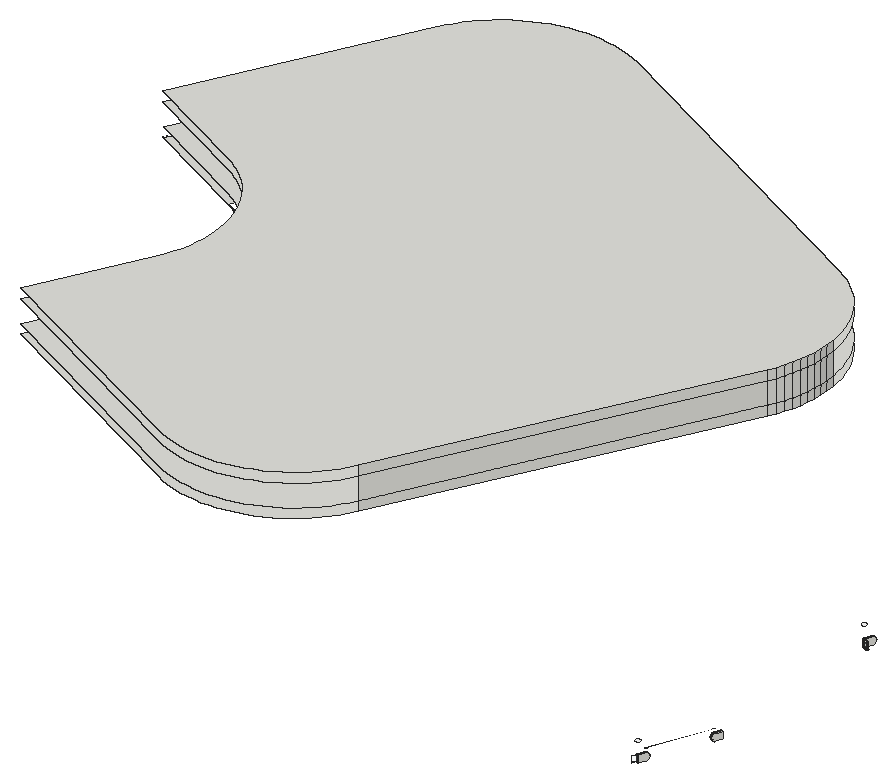
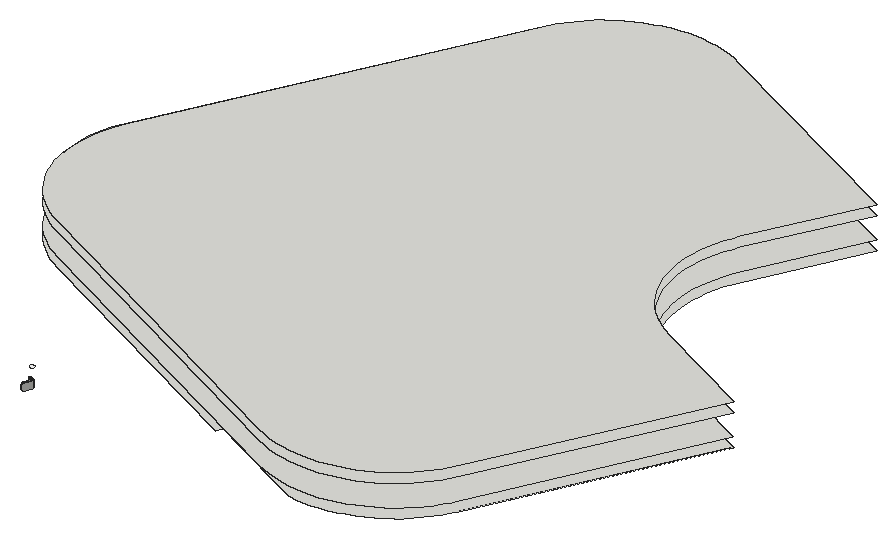
# SketchUp Ruby script. Lengths in inches.
U = 1.inch
M = Sketchup.active_model
def pt(a) = Geom::Point3d.new(a.map { |v| v * U })
def face(e, loops, mat)
  f = e.add_face(loops[0].map { |a| pt(a) })
  loops[1..].each { |l| e.add_face(l.map { |a| pt(a) }).erase! }
  f.material = f.back_material = mat if mat
  f
end
# faces: each face lists its corners as indices into pts; further lists are holes
def faces(e, pts, list, mat = nil) = list.each { |f| face(e, (f[0].is_a?(Array) ? f : [f]).map { |l| l.map { |i| pts[i] } }, mat) }
# xy, xz, yz: faces in a plane at the given z, y or x. An outline is a flat list of corners, or four numbers for a rectangle; further outlines are holes
def ring(l) = l.size == 4 ? [[l[0], l[1]], [l[2], l[1]], [l[2], l[3]], [l[0], l[3]]] : l.each_slice(2).to_a
def flat(e, list, mat, &to3) = list.each { |f| face(e, (f[0].is_a?(Array) ? f : [f]).map { |l| ring(l).map { |u, v| to3.(u, v) } }, mat) }
def xy(e, z, list, mat = nil) = flat(e, list, mat) { |x, y| [x, y, z] }
def xz(e, y, list, mat = nil) = flat(e, list, mat) { |x, z| [x, y, z] }
def yz(e, x, list, mat = nil) = flat(e, list, mat) { |y, z| [x, y, z] }
def lines(e, pts, list) = list.each { |a, b| e.add_line(pt(pts[a]), pt(pts[b])) }
# prism: a flat outline (further loops are holes) pulled along v
def prism(e, loops, v, mat = nil)
  f = face(e, loops, mat); d = Geom::Vector3d.new(v.map { |x| x * U })
  f.pushpull(f.normal.samedirection?(d) ? d.length : -d.length)
end
def box(e, o, s, mat = nil) = prism(e, [[o, [o[0] + s[0], o[1], o[2]], [o[0] + s[0], o[1] + s[1], o[2]], [o[0], o[1] + s[1], o[2]]]], [0, 0, s[2]], mat)
def at(x, y, z, deg = 0) = Geom::Transformation.translation(pt([x, y, z])) * Geom::Transformation.rotation(ORIGIN, Z_AXIS, deg.degrees)
def axes(o, x, y, z) = Geom::Transformation.new([*x, 0, *y, 0, *z, 0, *pt(o).to_a, 1])
def part(name) = M.definitions.add(name)
# library, detail: a bought-in or finely detailed component or shape, given as its bounding box
def library(name, o, s) = part(name).tap { |d| box(d.entities, o, s) }
def detail(e, o, s) = box(e.add_group.entities, o, s)
def put(e, d, t, mat = nil) = e.add_instance(d, t).tap { |i| i.material = mat if mat }
def group(e, t, mat = nil) = e.add_group.tap { |g| g.transformation = t; g.material = mat if mat }.entities
root = M.entities
M.materials.add("Glass_Safety_01").color = [204, 235, 244]
M.materials["Glass_Safety_01"].alpha = 0.1
M.materials.add("[Color_000]").color = [255, 255, 255]
xy(root,351.283,[[955.297,790.187,955.04,790.287,955.76,792.12,956.016,792.019],[954.857,790.359,954.6,790.46,954.605,790.472,954.611,790.484,954.86,790.366],[954.86,790.366,954.611,790.484,955.32,792.292,955.577,792.192],[962.61,810.093,962.354,810.194,963.074,812.026,963.33,811.925,962.671,810.249],[963.328,866.978,961.618,867.953,961.755,868.193,963.309,867.306,963.464,867.217],
  [963.562,867.388,963.406,867.477,962.17,868.183,962.28,868.437,963.698,867.627],[962.146,868.129,961.894,868.239,961.929,868.32,962.04,868.574,962.68,870.044,962.932,869.934,962.28,868.437,962.04,868.574,961.989,868.603,961.852,868.364,961.929,868.32,962.17,868.183],[962.17,868.183,961.929,868.32,962.04,868.574,962.28,868.437],[961.713,868.317,961.46,868.428,962.246,870.232,962.499,870.122],[961.929,868.32,961.852,868.364,961.989,868.603,962.04,868.574]])
xy(root,351.362,[[954.36,788.859,954.182,788.944,954.857,790.359,954.948,790.323,955.037,790.281],[955.04,790.287,954.948,790.323,954.86,790.366,955.433,791.825,955.616,791.753],[954.948,790.323,954.857,790.359,954.858,790.363,954.86,790.366],[963.122,867.412,961.755,868.193,961.803,868.278,961.894,868.239,961.929,868.32,963.22,867.583],[961.894,868.239,961.803,868.278,961.852,868.364,961.929,868.32],
  [961.803,868.278,961.713,868.317,962.342,869.761,962.522,869.683,961.929,868.32,961.852,868.364]],"Glass_Safety_01")
xy(root,353.33,[[954.36,788.859,955.037,790.281,954.948,790.323,954.857,790.359,954.182,788.944],[955.04,790.287,955.616,791.753,955.433,791.825,954.86,790.366,954.948,790.323],[954.948,790.323,954.86,790.366,954.858,790.363,954.857,790.359],[963.122,867.412,963.22,867.583,961.929,868.32,961.894,868.239,961.803,868.278,961.755,868.193],[961.894,868.239,961.929,868.32,961.852,868.364,961.803,868.278],
  [961.803,868.278,961.852,868.364,961.929,868.32,962.522,869.683,962.342,869.761,961.713,868.317]],"Glass_Safety_01")
xy(root,353.409,[[955.297,790.187,956.016,792.019,955.76,792.12,955.04,790.287],[954.857,790.359,954.86,790.366,954.611,790.484,954.605,790.472,954.6,790.46],[954.86,790.366,955.577,792.192,955.32,792.292,954.611,790.484],[962.61,810.093,962.671,810.249,963.33,811.925,963.074,812.026,962.354,810.194],[963.328,866.978,963.464,867.217,963.309,867.306,961.755,868.193,961.618,867.953],
  [962.146,868.129,962.17,868.183,961.929,868.32,961.852,868.364,961.989,868.603,962.04,868.574,962.28,868.437,962.932,869.934,962.68,870.044,962.04,868.574,961.929,868.32,961.894,868.239],[962.17,868.183,962.28,868.437,962.04,868.574,961.929,868.32],[961.713,868.317,962.499,870.122,962.246,870.232,961.46,868.428],[961.929,868.32,962.04,868.574,961.989,868.603,961.852,868.364]])
xy(root,354.511,[[955.76,792.12,962.671,810.249,955.577,792.192],[955.76,792.12,962.855,810.177,962.671,810.249]],"Glass_Safety_01")
xy(root,357.267,[[954.993,789.695,955.155,789.728,955.302,789.802,955.425,789.911,955.515,790.048,955.567,790.204,955.577,790.368,955.544,790.53,955.47,790.677,955.361,790.8,955.224,790.89,955.068,790.942,954.903,790.952,954.742,790.919,954.595,790.845,954.472,790.736,954.382,790.599,954.33,790.442,954.32,790.278,954.353,790.117,954.427,789.97,954.536,789.847,954.673,789.757,954.829,789.705],[961.848,867.65,962.009,867.683,962.157,867.757,962.279,867.866,962.37,868.003,962.422,868.159,962.432,868.323,962.399,868.484,962.325,868.631,962.216,868.754,962.079,868.845,961.922,868.897,961.758,868.907,961.597,868.873,961.45,868.8,961.327,868.691,961.237,868.553,961.185,868.397,961.175,868.233,961.208,868.072,961.282,867.925,961.391,867.802,961.528,867.712,961.684,867.66]],"[Color_000]")
xy(root,412.837,[[[862.815,738.526,860.46,738.588,858.115,738.805,855.788,739.175,853.491,739.695,851.232,740.366,849.022,741.182,846.871,742.141,777.884,775.639,793.609,808.023,794.568,810.175,795.384,812.385,796.054,814.643,796.575,816.941,796.945,819.267,797.161,821.613,797.224,823.968,797.132,826.322,796.887,828.665,796.489,830.987,795.94,833.278,795.243,835.528,794.399,837.728,793.414,839.868,792.291,841.938,791.035,843.931,789.651,845.838,788.145,847.65,786.524,849.359,784.795,850.959,782.965,852.442,781.042,853.803,779.034,855.034,776.949,856.132,744.842,871.723,776.516,936.952,776.255,937.079,744.581,871.849,744.565,871.857,776.004,936.603,776.255,937.079,777.102,938.6875,778.334,940.695,779.694,942.619,781.178,944.449,782.777,946.178,784.487,947.799,786.299,949.304,788.205,950.688,790.198,951.944,792.269,953.068,794.409,954.053,796.608,954.896,798.859,955.594,801.149,956.143,803.471,956.541,805.814,956.786,808.168,956.877,810.523,956.815,812.869,956.598,841.084,942.898,826.624,913.117,831.121,910.933,845.582,940.714,846.416,942.432,925.484,904.039,927.568,902.941,929.577,901.71,931.5,900.349,933.33,898.866,935.059,897.266,936.68,895.556,938.186,893.744,939.569,891.838,940.826,889.845,941.949,887.774,942.934,885.634,943.777,883.435,944.475,881.185,945.024,878.894,945.422,876.572,945.667,874.229,945.759,871.875,945.696,869.52,945.479,867.174,945.11,864.848,944.589,862.55,943.919,860.292,943.102,858.082,942.143,855.93,894.98,758.8,893.882,756.716,892.65,754.708,891.29,752.785,889.806,750.954,888.206,749.225,886.497,747.604,884.685,746.099,882.779,744.715,880.786,743.459,878.715,742.336,876.575,741.35,874.375,740.507,872.125,739.809,869.834,739.26,867.512,738.862,865.169,738.617],[780.848,854.239,812.287,918.985,808.388,920.878,776.949,856.132],[851.789,784.021,853.66,784.074,855.491,784.231,857.275,784.493,859.004,784.858,860.67,785.324,862.267,785.89,863.788,786.552,865.226,787.309,866.574,788.157,867.828,789.092,868.982,790.111,870.03,791.209,870.969,792.381,871.794,793.622,872.502,794.927,878.32,806.909,877.223,804.825,875.991,802.817,874.63,800.893,873.147,799.063,871.547,797.334,869.838,795.713,868.026,794.208,866.119,792.824,864.79,791.986,864.577,791.797,863.497,790.992,862.336,790.262,861.098,789.61,859.789,789.04,858.414,788.553,856.979,788.151,855.49,787.837,854.557,787.7,853.175,787.369,850.853,786.971,848.51,786.726,846.156,786.635,843.801,786.697,841.455,786.914,839.129,787.284,836.831,787.804,834.573,788.474,832.363,789.291,830.211,790.25,834.524,788.156,836.381,787.308,838.272,786.551,840.19,785.889,842.127,785.323,844.073,784.857,846.02,784.493,847.961,784.231,849.887,784.074]],[851.789,784.021,849.887,784.074,847.961,784.231,846.02,784.493,844.073,784.857,842.127,785.323,840.19,785.889,838.272,786.551,836.381,787.308,834.524,788.156,830.211,790.25,832.363,789.291,834.573,788.474,836.831,787.804,839.129,787.284,841.455,786.914,843.801,786.697,846.156,786.635,848.51,786.726,850.853,786.971,853.175,787.369,854.557,787.7,855.49,787.837,856.979,788.151,858.414,788.553,859.789,789.04,861.098,789.61,862.336,790.262,863.497,790.992,864.577,791.797,864.79,791.986,866.119,792.824,868.026,794.208,869.838,795.713,871.547,797.334,873.147,799.063,874.63,800.893,875.991,802.817,877.223,804.825,878.32,806.909,872.502,794.927,871.794,793.622,870.969,792.381,870.03,791.209,868.982,790.111,867.828,789.092,866.574,788.157,865.226,787.309,863.788,786.552,862.267,785.89,860.67,785.324,859.004,784.858,857.275,784.493,855.491,784.231,853.66,784.074]])
xy(root,415.758,[[862.815,738.526,860.46,738.588,858.115,738.805,855.788,739.175,853.491,739.695,851.232,740.366,849.022,741.182,846.871,742.141,777.884,775.639,793.609,808.023,794.568,810.175,795.384,812.385,796.054,814.643,796.575,816.941,796.945,819.267,797.161,821.613,797.224,823.968,797.132,826.322,796.887,828.665,796.489,830.987,795.94,833.278,795.243,835.528,794.399,837.728,793.414,839.868,792.291,841.938,791.035,843.931,789.651,845.838,788.145,847.65,786.524,849.359,784.795,850.959,782.965,852.442,781.042,853.803,779.034,855.034,776.949,856.132,744.842,871.723,776.516,936.952,776.255,937.079,777.102,938.6875,778.334,940.695,779.694,942.619,781.178,944.449,782.777,946.178,784.487,947.799,786.299,949.304,788.205,950.688,790.198,951.944,792.269,953.068,794.409,954.053,796.608,954.896,798.859,955.594,801.149,956.143,803.471,956.541,805.814,956.786,808.168,956.877,810.523,956.815,812.869,956.598,815.196,956.229,817.493,955.708,819.752,955.038,821.961,954.221,824.113,953.262,925.484,904.039,927.568,902.941,929.577,901.71,931.5,900.349,933.33,898.866,935.059,897.266,936.68,895.556,938.186,893.744,939.569,891.838,940.826,889.845,941.949,887.774,942.934,885.634,943.777,883.435,944.475,881.185,945.024,878.894,945.422,876.572,945.667,874.229,945.759,871.875,945.696,869.52,945.479,867.174,945.11,864.848,944.589,862.55,943.919,860.292,943.102,858.082,942.143,855.93,894.98,758.8,893.882,756.716,892.65,754.708,891.29,752.785,889.806,750.954,888.206,749.225,886.497,747.604,884.685,746.099,882.779,744.715,880.786,743.459,878.715,742.336,876.575,741.35,874.375,740.507,872.125,739.809,869.834,739.26,867.512,738.862,865.169,738.617]])
xy(root,422.51,[[862.815,738.526,860.46,738.588,858.115,738.805,855.788,739.175,853.491,739.695,851.232,740.366,849.022,741.182,846.871,742.141,777.884,775.639,793.609,808.023,794.568,810.175,795.384,812.385,796.054,814.643,796.575,816.941,796.945,819.267,797.161,821.613,797.224,823.968,797.132,826.322,796.887,828.665,796.489,830.987,795.94,833.278,795.243,835.528,794.399,837.728,793.414,839.868,792.291,841.938,791.035,843.931,789.651,845.838,788.145,847.65,786.524,849.359,784.795,850.959,782.965,852.442,781.042,853.803,779.034,855.034,776.949,856.132,744.565,871.857,776.004,936.603,777.102,938.6875,778.334,940.695,779.694,942.619,781.178,944.449,782.777,946.178,784.487,947.799,786.299,949.304,788.205,950.688,790.198,951.944,792.269,953.068,794.409,954.053,796.608,954.896,798.859,955.594,801.149,956.143,803.471,956.541,805.814,956.786,808.168,956.877,810.523,956.815,812.869,956.598,815.196,956.229,817.493,955.708,819.752,955.038,821.961,954.221,824.113,953.262,925.484,904.039,927.568,902.941,929.577,901.71,931.5,900.349,933.33,898.866,935.059,897.266,936.68,895.556,938.186,893.744,939.569,891.838,940.826,889.845,941.949,887.774,942.934,885.634,943.777,883.435,944.475,881.185,945.024,878.894,945.422,876.572,945.667,874.229,945.759,871.875,945.696,869.52,945.479,867.174,945.11,864.848,944.589,862.55,943.919,860.292,943.102,858.082,942.143,855.93,894.98,758.8,893.882,756.716,892.65,754.708,891.29,752.785,889.806,750.954,888.206,749.225,886.497,747.604,884.685,746.099,882.779,744.715,880.786,743.459,878.715,742.336,876.575,741.35,874.375,740.507,872.125,739.809,869.834,739.26,867.512,738.862,865.169,738.617]])
xy(root,425.526,[[862.815,738.526,865.169,738.617,867.512,738.862,869.834,739.26,872.125,739.809,874.375,740.507,876.575,741.35,878.715,742.336,880.786,743.459,882.779,744.715,884.685,746.099,886.497,747.604,888.206,749.225,889.806,750.954,891.29,752.785,892.65,754.708,893.882,756.716,894.98,758.8,942.143,855.93,943.102,858.082,943.919,860.292,944.589,862.55,945.11,864.848,945.479,867.174,945.696,869.52,945.759,871.875,945.667,874.229,945.422,876.572,945.024,878.894,944.475,881.185,943.777,883.435,942.934,885.634,941.949,887.774,940.826,889.845,939.569,891.838,938.186,893.744,936.68,895.556,935.059,897.266,933.33,898.866,931.5,900.349,929.577,901.71,927.568,902.941,925.484,904.039,824.113,953.262,821.961,954.221,819.752,955.038,817.493,955.708,815.196,956.229,812.869,956.598,810.523,956.815,808.168,956.877,805.814,956.786,803.471,956.541,801.149,956.143,798.859,955.594,796.608,954.896,794.409,954.053,792.269,953.068,790.198,951.944,788.205,950.688,786.299,949.304,784.487,947.799,782.777,946.178,781.178,944.449,779.694,942.619,778.334,940.695,777.102,938.6875,776.004,936.603,744.565,871.857,776.949,856.132,779.034,855.034,781.042,853.803,782.965,852.442,784.795,850.959,786.524,849.359,788.145,847.65,789.651,845.838,791.035,843.931,792.291,841.938,793.414,839.868,794.399,837.728,795.243,835.528,795.94,833.278,796.489,830.987,796.887,828.665,797.132,826.322,797.224,823.968,797.161,821.613,796.945,819.267,796.575,816.941,796.054,814.643,795.384,812.385,794.568,810.175,793.609,808.023,777.884,775.639,846.871,742.141,849.022,741.182,851.232,740.366,853.491,739.695,855.788,739.175,858.115,738.805,860.46,738.588]])
p = [[955.037,790.281,351.283],[955.037,790.281,351.362],[955.037,790.281,353.33],[955.037,790.281,353.409],[955.286,790.162,353.409],[955.286,790.162,351.283],
  [955.04,790.287,351.362],[955.04,790.287,351.283],[955.297,790.187,351.283],[955.297,790.187,353.409],[955.04,790.287,353.409],[955.04,790.287,353.33],
  [956.016,792.019,353.409],[956.016,792.019,351.283],[956.117,792.275,351.319],[956.211,792.513,351.425],[956.291,792.718,351.594],[956.353,792.876,351.814],
  [956.392,792.974,352.071],[956.405,793.008,352.346],[956.392,792.974,352.621],[956.353,792.876,352.877],[956.291,792.718,353.098],[956.211,792.513,353.267],
  [956.117,792.275,353.373],[955.76,792.12,353.409],[955.76,792.12,351.283],[955.616,791.753,351.362],[955.616,791.753,353.33],[954.857,790.359,351.283],
  [954.857,790.359,351.362],[954.857,790.359,353.33],[954.857,790.359,353.409],[954.6,790.46,353.409],[954.6,790.46,351.283],[954.86,790.366,351.362],
  [954.86,790.366,351.283],[954.611,790.484,351.283],[954.611,790.484,353.409],[954.86,790.366,353.409],[954.86,790.366,353.33],[955.577,792.192,351.283],
  [955.677,792.448,351.319],[955.771,792.686,351.425],[955.852,792.891,351.594],[955.913,793.048,351.814],[955.952,793.147,352.071],[955.965,793.181,352.346],
  [955.952,793.147,352.621],[955.913,793.048,352.877],[955.852,792.891,353.098],[955.771,792.686,353.267],[955.677,792.448,353.373],[955.577,792.192,353.409],
  [954.605,790.472,351.283],[954.605,790.472,353.409],[955.32,792.292,353.409],[955.421,792.548,353.373],[955.515,792.787,353.267],[955.595,792.992,353.098],
  [955.657,793.149,352.877],[955.696,793.248,352.621],[955.709,793.282,352.346],[955.696,793.248,352.071],[955.657,793.149,351.814],[955.595,792.992,351.594],
  [955.515,792.787,351.425],[955.421,792.548,351.319],[955.32,792.292,351.283],[955.86,792.376,351.319],[955.954,792.614,351.425],[956.035,792.819,351.594],
  [956.097,792.976,351.814],[956.135,793.075,352.071],[956.149,793.109,352.346],[956.135,793.075,352.621],[956.097,792.976,352.877],[956.035,792.819,353.098],
  [955.954,792.614,353.267],[955.86,792.376,353.373],[963.05,809.92,351.283],[963.765,811.74,351.283],[963.765,811.74,353.409],[963.05,809.92,353.409],
  [962.949,809.664,353.373],[962.856,809.426,353.267],[962.775,809.221,353.098],[962.713,809.064,352.877],[962.675,808.965,352.621],[962.661,808.931,352.346],
  [962.675,808.965,352.071],[962.713,809.064,351.814],[962.775,809.221,351.594],[962.856,809.426,351.425],[962.949,809.664,351.319],[962.855,810.177,353.409],
  [963.512,811.85,353.409],[963.512,811.85,353.33],[963.512,811.85,351.362],[963.512,811.85,351.283],[962.855,810.177,351.283],[962.794,810.021,351.283],
  [962.693,809.765,351.319],[962.599,809.527,351.425],[962.519,809.322,351.594],[962.457,809.164,351.814],[962.418,809.066,352.071],[962.405,809.032,352.346],
  [962.418,809.066,352.621],[962.457,809.164,352.877],[962.519,809.322,353.098],[962.599,809.527,353.267],[962.693,809.765,353.373],[962.794,810.021,353.409],
  [962.61,810.093,351.283],[962.671,810.249,351.283],[962.671,810.249,353.409],[962.61,810.093,353.409],[962.51,809.837,353.373],[962.416,809.599,353.267],
  [962.335,809.394,353.098],[962.274,809.236,352.877],[962.235,809.138,352.621],[962.222,809.104,352.346],[962.235,809.138,352.071],[962.274,809.236,351.814],
  [962.335,809.394,351.594],[962.416,809.599,351.425],[962.51,809.837,351.319],[962.354,810.194,353.409],[963.074,812.026,353.409],[963.074,812.026,351.283],
  [962.354,810.194,351.283],[962.253,809.938,351.319],[962.159,809.699,351.425],[962.079,809.494,351.594],[962.017,809.337,351.814],[961.978,809.238,352.071],
  [961.965,809.205,352.346],[961.978,809.238,352.621],[962.017,809.337,352.877],[962.079,809.494,353.098],[962.159,809.699,353.267],[962.253,809.938,353.373],
  [963.33,811.925,353.409],[963.33,811.925,351.283],[963.33,811.925,351.362],[962.754,810.46,351.362],[962.754,810.46,353.33],[963.33,811.925,353.33],
  [961.755,868.193,353.409],[963.309,867.306,353.409],[963.309,867.306,351.283],[961.755,868.193,351.283],[961.755,868.193,351.362],[963.122,867.412,351.362],
  [963.122,867.412,353.33],[961.755,868.193,353.33],[962.17,868.183,351.283],[963.406,867.477,351.283],[963.406,867.477,353.409],[962.17,868.183,353.409],
  [961.929,868.32,353.409],[961.852,868.364,353.409],[961.852,868.364,353.33],[961.929,868.32,353.33],[963.22,867.583,353.33],[963.22,867.583,351.362],
  [961.929,868.32,351.362],[961.852,868.364,351.362],[961.852,868.364,351.283],[961.929,868.32,351.283],[961.618,867.953,351.283],[961.618,867.953,353.409],
  [961.894,868.239,351.362],[961.894,868.239,351.283],[962.146,868.129,351.283],[962.146,868.129,353.409],[961.894,868.239,353.409],[961.894,868.239,353.33],
  [962.28,868.437,351.283],[962.932,869.934,351.283],[963.042,870.186,351.319],[963.145,870.421,351.425],[963.232,870.623,351.594],[963.3,870.778,351.814],
  [963.342,870.875,352.071],[963.357,870.908,352.346],[963.342,870.875,352.621],[963.3,870.778,352.877],[963.232,870.623,353.098],[963.145,870.421,353.267],
  [963.042,870.186,353.373],[962.932,869.934,353.409],[962.28,868.437,353.409],[962.04,868.574,353.409],[962.68,870.044,353.409],[962.68,870.044,351.283],
  [962.04,868.574,351.283],[962.522,869.683,351.362],[962.522,869.683,353.33],[961.713,868.317,351.283],[961.713,868.317,351.362],[961.713,868.317,353.33],
  [961.713,868.317,353.409],[961.46,868.428,353.409],[961.46,868.428,351.283],[962.499,870.122,351.283],[962.499,870.122,353.409],[962.342,869.761,353.33],
  [962.342,869.761,351.362],[962.246,870.232,353.409],[962.356,870.485,353.373],[962.459,870.72,353.267],[962.547,870.921,353.098],[962.614,871.076,352.877],
  [962.656,871.174,352.621],[962.671,871.207,352.346],[962.656,871.174,352.071],[962.614,871.076,351.814],[962.547,870.921,351.594],[962.459,870.72,351.425],
  [962.356,870.485,351.319],[962.246,870.232,351.283],[961.989,868.603,353.409],[961.989,868.603,351.283],[962.789,870.296,351.319],[962.892,870.531,351.425],
  [962.98,870.733,351.594],[963.047,870.888,351.814],[963.09,870.985,352.071],[963.104,871.018,352.346],[963.09,870.985,352.621],[963.047,870.888,352.877],
  [962.98,870.733,353.098],[962.892,870.531,353.267],[962.789,870.296,353.373],[962.609,870.374,351.319],[962.609,870.374,353.373],[962.711,870.61,353.267],
  [962.799,870.811,353.098],[962.867,870.966,352.877],[962.909,871.064,352.621],[962.924,871.097,352.346],[962.909,871.064,352.071],[962.867,870.966,351.814],
  [962.799,870.811,351.594],[962.711,870.61,351.425],[954.182,788.944,353.33],[954.182,788.944,351.362],[954.948,790.323,351.362],[954.948,790.323,353.33],
  [954.858,790.363,353.33],[954.858,790.363,351.362],[955.433,791.825,351.362],[955.433,791.825,353.33],[962.9375,810.388,351.362],[962.9375,810.388,353.33],
  [961.803,868.278,353.33],[961.803,868.278,351.362],[894.98,758.8,412.837],[942.143,855.93,412.837],[942.143,855.93,415.758],[894.98,758.8,415.758],
  [943.102,858.082,412.837],[943.102,858.082,415.758],[943.919,860.292,412.837],[943.919,860.292,415.758],[944.589,862.55,412.837],[944.589,862.55,415.758],
  [945.11,864.848,412.837],[945.11,864.848,415.758],[945.479,867.174,412.837],[945.479,867.174,415.758],[945.696,869.52,412.837],[945.696,869.52,415.758],
  [945.759,871.875,412.837],[945.759,871.875,415.758],[945.667,874.229,412.837],[945.667,874.229,415.758],[945.422,876.572,412.837],[945.422,876.572,415.758],
  [942.143,855.93,422.51],[894.98,758.8,422.51],[943.102,858.082,422.51],[943.919,860.292,422.51],[944.589,862.55,422.51],[945.11,864.848,422.51],
  [945.479,867.174,422.51],[945.696,869.52,422.51],[945.759,871.875,422.51],[945.667,874.229,422.51],[945.422,876.572,422.51],[942.143,855.93,425.526],
  [894.98,758.8,425.526],[943.102,858.082,425.526],[943.919,860.292,425.526],[944.589,862.55,425.526],[945.11,864.848,425.526],[945.479,867.174,425.526],
  [945.696,869.52,425.526],[945.759,871.875,425.526],[945.667,874.229,425.526],[945.422,876.572,425.526]]
faces(root,p,[[0,1,2,3,4,5],[6,7,8,9,10,11],[12,9,8,13,14,15,16,17,18,19,20,21,22,23,24],[10,25,26,7,6,27,28,11],[29,30,31,32,33,34],[35,36,37,38,39,40],[39,32,31,30,29,36,35,40],[39,32,31,30,29,36,41,42,43,44,45,46,47,48,49,50,51,52,53],
  [54,34,33,55,38,37],[33,55,38,56,57,58,59,60,61,62,63,64,65,66,67,68,37,54,34],[26,69,14,13],[42,41,68,67],[69,70,15,14],[43,42,67,66],[80,81,82,83,84,85,86,87,88,89,90,91,92,93,94],[95,96,97,98,99,100,101,102,103,104,105,106,107,108,109,110,111,112,113],
  [114,115,116,117,118,119,120,121,122,123,124,125,126,127,128],[129,130,131,132,133,134,135,136,137,138,139,140,141,142,143],[103,102,94,93],[128,127,134,133],[102,101,80,94],[114,128,133,132],[144,116,115,145,146,147,148,149],[150,151,152,153,154,155,156,157],
  [158,159,160,161,162,163,164,165,166,167,168,169,170,171],[154,153,172,173,150,157],[174,175,176,177,178,179],[161,177,176,158,180,181,182,183,184,185,186,187,188,189,190,191,192,193,194],[195,196,197,198,171,175,174,168,199,200,165,179,178,162],[201,202,203,204,205,206],[201,207,208,204,203,209,210,202],[205,211,212,213,214,215,216,217,218,219,220,221,222,223,206],
  [170,169,164,163,224,225],[197,226,182,181],[237,207,223,222],[226,227,183,182],[247,237,222,221],[70,71,16,15],[44,43,66,65],[104,103,93,92],
  [127,126,135,134],[246,247,221,220],[71,72,17,16],[45,44,65,64],[105,104,92,91],[126,125,136,135],[245,246,220,219],[72,73,18,17],
  [46,45,64,63],[106,105,91,90],[125,124,137,136],[244,245,219,218],[73,74,19,18],[47,46,63,62],[107,106,90,89],[124,123,138,137],
  [243,244,218,217],[74,75,20,19],[48,47,62,61],[108,107,89,88],[123,122,139,138],[242,243,217,216],[75,76,21,20],[49,48,61,60],
  [109,108,88,87],[122,121,140,139],[241,242,216,215],[76,77,22,21],[50,49,60,59],[110,109,87,86],[121,120,141,140],[240,241,215,214],
  [77,78,23,22],[51,50,59,58],[111,110,86,85],[120,119,142,141],[239,240,214,213],[78,79,24,23],[52,51,58,57],[112,111,85,84],
  [119,118,143,142],[235,236,192,191],[238,239,213,212],[79,25,12,24],[53,52,57,56],[113,112,84,83],[118,117,129,143],[236,196,193,192],
  [208,238,212,211],[260,261,262,263],[264,265,262,261],[266,267,265,264],[268,269,267,266],[270,271,269,268],[272,273,271,270],[274,275,273,272],
  [276,277,275,274],[278,279,277,276],[280,281,279,278],[263,262,282,283],[262,265,284,282],[265,267,285,284],[267,269,286,285],[269,271,287,286],
  [271,273,288,287],[273,275,289,288],[275,277,290,289],[277,279,291,290],[279,281,292,291],[283,282,293,294],[282,284,295,293],[284,285,296,295],
  [285,286,297,296],[286,287,298,297],[287,288,299,298],[288,289,300,299],[289,290,301,300],[290,291,302,301],[291,292,303,302]])
faces(root,p,[[25,26,69,70,71,72,73,74,75,76,77,78,79],[41,53,52,51,50,49,48,47,46,45,44,43,42],[196,197,226,227,228,229,230,231,232,233,234,235,236],[207,208,238,239,240,241,242,243,244,245,246,247,237],[248,31,30,249],[1,250,251,2],[251,250,6,11],[250,251,31,30],
  [40,251,250,35],[11,28,27,6],[252,40,35,253,30,31],[254,35,40,255],[27,254,255,28],[148,147,256,257],[157,156,155,154],[165,164,169,168,167,166],
  [157,258,259,154],[258,259,174,179],[179,165,200,199,168,174],[259,258,203,202],[209,203,202,210],[169,259,258,164],[209,200,199,210]],"Glass_Safety_01")
